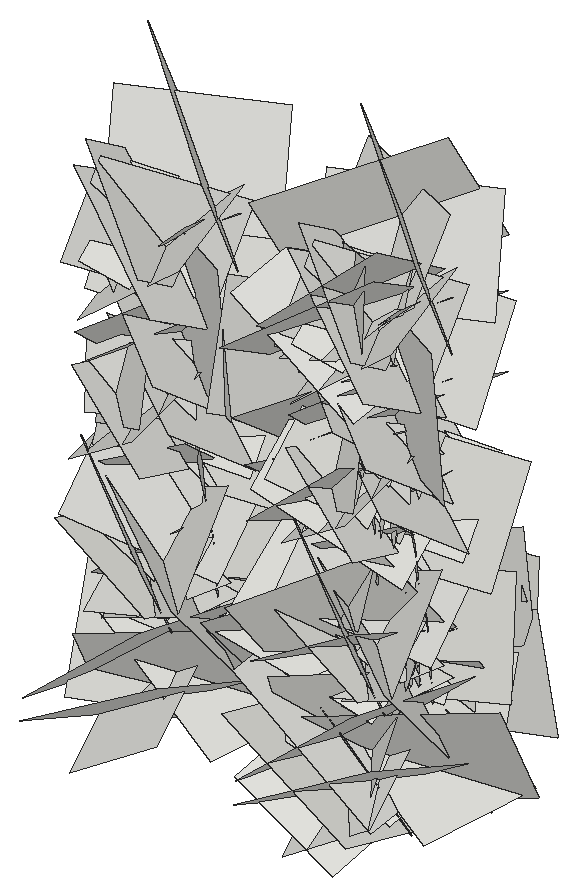
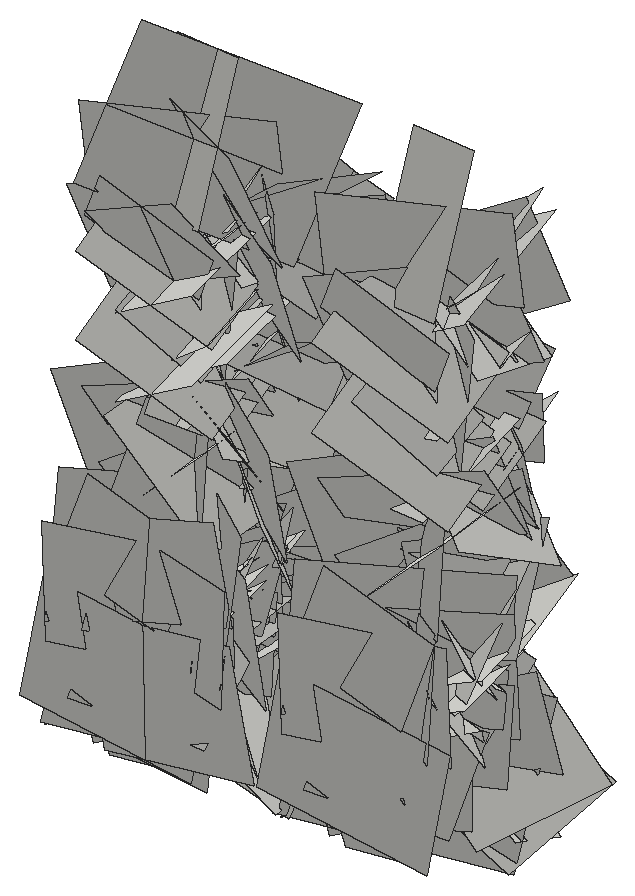
# SketchUp Ruby script. Lengths in inches.
U = 1.inch
M = Sketchup.active_model
def pt(a) = Geom::Point3d.new(a.map { |v| v * U })
def face(e, loops, mat)
  f = e.add_face(loops[0].map { |a| pt(a) })
  loops[1..].each { |l| e.add_face(l.map { |a| pt(a) }).erase! }
  f.material = f.back_material = mat if mat
  f
end
# faces: each face lists its corners as indices into pts; further lists are holes
def faces(e, pts, list, mat = nil) = list.each { |f| face(e, (f[0].is_a?(Array) ? f : [f]).map { |l| l.map { |i| pts[i] } }, mat) }
# xy, xz, yz: faces in a plane at the given z, y or x. An outline is a flat list of corners, or four numbers for a rectangle; further outlines are holes
def ring(l) = l.size == 4 ? [[l[0], l[1]], [l[2], l[1]], [l[2], l[3]], [l[0], l[3]]] : l.each_slice(2).to_a
def flat(e, list, mat, &to3) = list.each { |f| face(e, (f[0].is_a?(Array) ? f : [f]).map { |l| ring(l).map { |u, v| to3.(u, v) } }, mat) }
def xy(e, z, list, mat = nil) = flat(e, list, mat) { |x, y| [x, y, z] }
def xz(e, y, list, mat = nil) = flat(e, list, mat) { |x, z| [x, y, z] }
def yz(e, x, list, mat = nil) = flat(e, list, mat) { |y, z| [x, y, z] }
def lines(e, pts, list) = list.each { |a, b| e.add_line(pt(pts[a]), pt(pts[b])) }
# prism: a flat outline (further loops are holes) pulled along v
def prism(e, loops, v, mat = nil)
  f = face(e, loops, mat); d = Geom::Vector3d.new(v.map { |x| x * U })
  f.pushpull(f.normal.samedirection?(d) ? d.length : -d.length)
end
def box(e, o, s, mat = nil) = prism(e, [[o, [o[0] + s[0], o[1], o[2]], [o[0] + s[0], o[1] + s[1], o[2]], [o[0], o[1] + s[1], o[2]]]], [0, 0, s[2]], mat)
def at(x, y, z, deg = 0) = Geom::Transformation.translation(pt([x, y, z])) * Geom::Transformation.rotation(ORIGIN, Z_AXIS, deg.degrees)
def axes(o, x, y, z) = Geom::Transformation.new([*x, 0, *y, 0, *z, 0, *pt(o).to_a, 1])
def part(name) = M.definitions.add(name)
# library, detail: a bought-in or finely detailed component or shape, given as its bounding box
def library(name, o, s) = part(name).tap { |d| box(d.entities, o, s) }
def detail(e, o, s) = box(e.add_group.entities, o, s)
def put(e, d, t, mat = nil) = e.add_instance(d, t).tap { |i| i.material = mat if mat }
def group(e, t, mat = nil) = e.add_group.tap { |g| g.transformation = t; g.material = mat if mat }.entities
root = M.entities
c1 = part("Component\#6")
p = [[0.01,0,0],[0,3.24,4.54],[4.32,3.24,4.54],[4.33,0,0]]
faces(c1.entities,p,[[0,1,2,3]])
put(root,c1,axes([424.49,208.64,6.82],[-0.0498,0.28937,-0.67344],[-0.06797,-0.67386,-0.28508],[-0.77398,0.04056,0.06836]))
put(root,c1,axes([410.71,210.125,0.49],[0.19083,-0.77607,-0.35788],[0.04853,-0.35645,0.796],[0.90459,0.18284,0.03279]))
put(root,c1,axes([424.49,210.125,0.49],[-0.19083,-0.77607,-0.35788],[-0.04853,-0.35645,0.796],[-0.90459,0.18284,0.03279]))
put(root,c1,axes([420.52,210.125,0.49],[0.19083,-0.77607,-0.35788],[0.04853,-0.35645,0.796],[0.90459,0.18284,0.03279]))
put(root,c1,axes([410.71,210.53,-0.53],[-0.13793,-1.11303,0.36033],[0.12678,0.348,1.11812],[1.23359,-0.16021,-0.07463]))
put(root,c1,axes([424.49,210.53,-0.53],[0.13793,-1.11303,0.36033],[-0.12678,0.348,1.11812],[-1.23359,-0.16021,-0.07463]))
put(root,c1,axes([420.52,210.53,-0.53],[-0.13793,-1.11303,0.36033],[0.12678,0.348,1.11812],[1.23359,-0.16021,-0.07463]))
put(root,c1,axes([410.71,209.89,15.21],[0.14915,-0.31655,-0.61374],[0.00846,-0.62556,0.32448],[0.73195,0.07174,0.12131]))
put(root,c1,axes([424.49,209.89,15.21],[-0.14915,-0.31655,-0.61374],[-0.00846,-0.62556,0.32448],[-0.73195,0.07174,0.12131]))
put(root,c1,axes([420.52,209.89,15.21],[0.14915,-0.31655,-0.61374],[0.00846,-0.62556,0.32448],[0.73195,0.07174,0.12131]))
put(root,c1,axes([414.68,209.73,11.28],[0.10776,-0.78869,0.28769],[0.10217,0.29884,0.7852],[-0.88401,-0.0616,0.12582]))
put(root,c1,axes([420.52,209.73,11.28],[-0.10776,-0.78869,0.28769],[-0.10217,0.29884,0.7852],[0.88401,-0.0616,0.12582]))
put(root,c1,axes([424.49,209.73,11.28],[0.10776,-0.78869,0.28769],[0.10217,0.29884,0.7852],[-0.88401,-0.0616,0.12582]))
put(root,c1,axes([424.49,208.44,11.85],[0.18719,0.63062,-0.8853],[0.07209,-0.90156,-0.62864],[-1.1499,0.04614,-0.18352]))
put(root,c1,axes([410.71,208.44,11.85],[-0.18719,0.63062,-0.8853],[-0.07209,-0.90156,-0.62864],[1.1499,0.04614,-0.18352]))
put(root,c1,axes([420.52,208.44,11.85],[-0.18719,0.63062,-0.8853],[-0.07209,-0.90156,-0.62864],[1.1499,0.04614,-0.18352]))
put(root,c1,axes([410.71,206.93,9.09],[-0.09893,0.82066,-0.28112],[0.08874,-0.2729,-0.82446],[0.91523,0.11517,0.04956]))
put(root,c1,axes([424.49,206.93,9.09],[0.09893,0.82066,-0.28112],[-0.08874,-0.2729,-0.82446],[-0.91523,0.11517,0.04956]))
put(root,c1,axes([420.52,206.93,9.09],[-0.09893,0.82066,-0.28112],[0.08874,-0.2729,-0.82446],[0.91523,0.11517,0.04956]))
put(root,c1,axes([414.68,210.2,16.34],[0.08816,-0.12898,-0.67949],[-0.09646,-0.68047,0.11803],[-0.72675,0.07467,-0.09809]))
put(root,c1,axes([420.52,210.2,16.34],[-0.08816,-0.12898,-0.67949],[0.09646,-0.68047,0.11803],[0.72675,0.07467,-0.09809]))
put(root,c1,axes([424.49,210.2,16.34],[0.08816,-0.12898,-0.67949],[-0.09646,-0.68047,0.11803],[-0.72675,0.07467,-0.09809]))
put(root,c1,axes([414.68,208.78,18.92],[-0.08317,0.53287,-0.42892],[0.0846,-0.42165,-0.53844],[-0.72013,-0.11108,-0.01372]))
put(root,c1,axes([420.52,208.78,18.92],[0.08317,0.53287,-0.42892],[-0.0846,-0.42165,-0.53844],[0.72013,-0.11108,-0.01372]))
put(root,c1,axes([424.49,208.78,18.92],[-0.08317,0.53287,-0.42892],[0.0846,-0.42165,-0.53844],[-0.72013,-0.11108,-0.01372]))
put(root,c1,axes([410.71,212.18,1.04],[-0.25647,-1.30664,0.09966],[-0.13645,0.12456,1.32049],[1.38234,-0.23013,0.14883]))
put(root,c1,axes([424.49,212.18,1.04],[0.25647,-1.30664,0.09966],[0.13645,0.12456,1.32049],[-1.38234,-0.23013,0.14883]))
put(root,c1,axes([420.52,212.18,1.04],[-0.25647,-1.30664,0.09966],[-0.13645,0.12456,1.32049],[1.38234,-0.23013,0.14883]))
put(root,c1,axes([410.71,208.07,23.15],[0.06368,1.0247,-0.55961],[-0.10104,-0.55418,-1.02498],[1.23347,-0.0983,-0.05507]))
put(root,c1,axes([424.49,208.07,23.15],[-0.06368,1.0247,-0.55961],[0.10104,-0.55418,-1.02498],[-1.23347,-0.0983,-0.05507]))
put(root,c1,axes([420.52,208.07,23.15],[0.06368,1.0247,-0.55961],[-0.10104,-0.55418,-1.02498],[1.23347,-0.0983,-0.05507]))
put(root,c1,axes([414.68,211.39,19.29],[0.15412,-0.67583,-0.24542],[-0.06417,-0.26101,0.68288],[-0.75944,-0.11509,-0.10751]))
put(root,c1,axes([420.52,211.39,19.29],[-0.15412,-0.67583,-0.24542],[0.06417,-0.26101,0.68288],[0.75944,-0.11509,-0.10751]))
put(root,c1,axes([424.49,211.39,19.29],[0.15412,-0.67583,-0.24542],[-0.06417,-0.26101,0.68288],[-0.75944,-0.11509,-0.10751]))
put(root,c1,axes([414.68,210.2,18.35],[0.0434,-0.8468,0.50557],[0.21084,0.5027,0.82588],[-1.02393,0.06762,0.19149]))
put(root,c1,axes([420.52,210.2,18.35],[-0.0434,-0.8468,0.50557],[-0.21084,0.5027,0.82588],[1.02393,0.06762,0.19149]))
put(root,c1,axes([424.49,210.2,18.35],[0.0434,-0.8468,0.50557],[0.21084,0.5027,0.82588],[-1.02393,0.06762,0.19149]))
put(root,c1,axes([410.71,211.18,6.7],[0.06152,-0.66215,-0.45123],[0.20693,-0.42709,0.65185],[0.82377,0.15673,-0.13005]))
put(root,c1,axes([424.49,211.18,6.7],[-0.06152,-0.66215,-0.45123],[-0.20693,-0.42709,0.65185],[-0.82377,0.15673,-0.13005]))
put(root,c1,axes([420.52,211.18,6.7],[0.06152,-0.66215,-0.45123],[0.20693,-0.42709,0.65185],[0.82377,0.15673,-0.13005]))
put(root,c1,axes([410.71,209.17,10.9],[-0.01303,0.87895,-0.98683],[-0.04513,-0.98662,-0.87824],[1.40007,-0.02362,-0.03749]))
put(root,c1,axes([424.49,209.17,10.9],[0.01303,0.87895,-0.98683],[0.04513,-0.98662,-0.87824],[-1.40007,-0.02362,-0.03749]))
put(root,c1,axes([420.52,209.17,10.9],[-0.01303,0.87895,-0.98683],[-0.04513,-0.98662,-0.87824],[1.40007,-0.02362,-0.03749]))
put(root,c1,axes([410.71,212.1,18.5625],[0.14567,-1.06407,-0.312],[-0.08976,-0.32354,1.06612],[1.17197,0.10748,0.12044]))
put(root,c1,axes([424.49,212.1,18.5625],[-0.14567,-1.06407,-0.312],[0.08976,-0.32354,1.06612],[-1.17197,0.10748,0.12044]))
put(root,c1,axes([420.52,212.1,18.5625],[0.14567,-1.06407,-0.312],[-0.08976,-0.32354,1.06612],[1.17197,0.10748,0.12044]))
put(root,c1,axes([410.71,212.58,7.86],[0.11208,-0.8157,-0.84783],[-0.04176,-0.85323,0.81597],[1.2464,0.04476,0.10358]))
put(root,c1,axes([424.49,212.58,7.86],[-0.11208,-0.8157,-0.84783],[0.04176,-0.85323,0.81597],[-1.2464,0.04476,0.10358]))
put(root,c1,axes([420.52,212.58,7.86],[0.11208,-0.8157,-0.84783],[-0.04176,-0.85323,0.81597],[1.2464,0.04476,0.10358]))
put(root,c1,axes([410.71,213.11,12.64],[-0.17797,-1.01022,-0.50589],[-0.14692,-0.48916,1.02282],[1.18855,-0.21174,0.05069]))
put(root,c1,axes([424.49,213.11,12.64],[0.17797,-1.01022,-0.50589],[0.14692,-0.48916,1.02282],[-1.18855,-0.21174,0.05069]))
put(root,c1,axes([420.52,213.11,12.64],[-0.17797,-1.01022,-0.50589],[-0.14692,-0.48916,1.02282],[1.18855,-0.21174,0.05069]))
put(root,c1,axes([424.49,207.33,19.43],[-0.19308,0.28824,0.9525],[0.12727,0.96762,-0.26985],[-1.04716,0.06445,-0.20842]))
put(root,c1,axes([410.71,207.33,19.43],[0.19308,0.28824,0.9525],[-0.12727,0.96762,-0.26985],[1.04716,0.06445,-0.20842]))
put(root,c1,axes([420.52,207.33,19.43],[0.19308,0.28824,0.9525],[-0.12727,0.96762,-0.26985],[1.04716,0.06445,-0.20842]))
put(root,c1,axes([410.71,209.23,19.24],[0.2079,0.89177,-0.6436],[-0.06754,-0.64344,-0.91097],[1.16379,-0.19665,0.06211]))
put(root,c1,axes([424.49,209.23,19.24],[-0.2079,0.89177,-0.6436],[0.06754,-0.64344,-0.91097],[-1.16379,-0.19665,0.06211]))
put(root,c1,axes([420.52,209.23,19.24],[0.2079,0.89177,-0.6436],[-0.06754,-0.64344,-0.91097],[1.16379,-0.19665,0.06211]))
put(root,c1,axes([414.68,209.48,12.42],[-0.00847,0.47556,-0.37402],[-0.05873,-0.37306,-0.47315],[-0.63863,0.028,0.04848]))
put(root,c1,axes([420.52,209.48,12.42],[0.00847,0.47556,-0.37402],[0.05873,-0.37306,-0.47315],[0.63863,0.028,0.04848]))
put(root,c1,axes([424.49,209.48,12.42],[-0.00847,0.47556,-0.37402],[-0.05873,-0.37306,-0.47315],[-0.63863,0.028,0.04848]))
put(root,c1,axes([410.71,207.16,9.13],[0.13241,0.57393,0.92472],[-0.131,0.93225,-0.56191],[1.14619,0.04024,-0.17105]))
put(root,c1,axes([424.49,207.16,9.13],[-0.13241,0.57393,0.92472],[0.131,0.93225,-0.56191],[-1.14619,0.04024,-0.17105]))
put(root,c1,axes([420.52,207.16,9.13],[0.13241,0.57393,0.92472],[-0.131,0.93225,-0.56191],[1.14619,0.04024,-0.17105]))
put(root,c1,axes([410.71,212.32,20.17],[0.18703,-0.0568,-1.36224],[0.02248,-1.37332,0.06001],[1.44505,0.02871,0.17537]))
put(root,c1,axes([424.49,212.32,20.17],[-0.18703,-0.0568,-1.36224],[-0.02248,-1.37332,0.06001],[-1.44505,0.02871,0.17537]))
put(root,c1,axes([420.52,212.32,20.17],[0.18703,-0.0568,-1.36224],[0.02248,-1.37332,0.06001],[1.44505,0.02871,0.17537]))
put(root,c1,axes([414.68,211.74,12.76],[-0.12736,-0.0958,-0.74557],[0.10526,-0.75044,0.08042],[-0.78982,-0.08457,0.13094]))
put(root,c1,axes([420.52,211.74,12.76],[0.12736,-0.0958,-0.74557],[-0.10526,-0.75044,0.08042],[0.78982,-0.08457,0.13094]))
put(root,c1,axes([424.49,211.74,12.76],[-0.12736,-0.0958,-0.74557],[0.10526,-0.75044,0.08042],[-0.78982,-0.08457,0.13094]))
put(root,c1,axes([410.71,209.9375,16.21],[0.25577,0.83815,-0.61941],[0.04278,-0.64283,-0.85412],[1.10389,-0.16928,0.17662]))
put(root,c1,axes([424.49,209.9375,16.21],[-0.25577,0.83815,-0.61941],[-0.04278,-0.64283,-0.85412],[-1.10389,-0.16928,0.17662]))
put(root,c1,axes([420.52,209.9375,16.21],[0.25577,0.83815,-0.61941],[0.04278,-0.64283,-0.85412],[1.10389,-0.16928,0.17662]))
put(root,c1,axes([410.71,210.25,-0.65],[0.14226,-0.69765,1.16631],[0.2044,1.1699,0.67761],[1.42601,-0.0981,-0.21348]))
put(root,c1,axes([424.49,210.25,-0.65],[-0.14226,-0.69765,1.16631],[-0.2044,1.1699,0.67761],[-1.42601,-0.0981,-0.21348]))
put(root,c1,axes([420.52,210.25,-0.65],[0.14226,-0.69765,1.16631],[0.2044,1.1699,0.67761],[1.42601,-0.0981,-0.21348]))
put(root,c1,axes([424.49,208.82,8.26],[0.05727,0.78185,-0.16779],[-0.14528,-0.15663,-0.77398],[-0.83509,0.08087,0.12314]))
put(root,c1,axes([410.71,208.82,8.26],[-0.05727,0.78185,-0.16779],[0.14528,-0.15663,-0.77398],[0.83509,0.08087,0.12314]))
put(root,c1,axes([420.52,208.82,8.26],[-0.05727,0.78185,-0.16779],[0.14528,-0.15663,-0.77398],[0.83509,0.08087,0.12314]))
put(root,c1,axes([410.71,211.87,13.61],[0.09122,-0.87293,0.35057],[-0.03759,0.34878,0.87716],[0.99643,0.09307,0.001]))
put(root,c1,axes([424.49,211.87,13.61],[-0.09122,-0.87293,0.35057],[0.03759,0.34878,0.87716],[-0.99643,0.09307,0.001]))
put(root,c1,axes([420.52,211.87,13.61],[0.09122,-0.87293,0.35057],[-0.03759,0.34878,0.87716],[0.99643,0.09307,0.001]))
put(root,c1,axes([414.68,210.23,8.89],[-0.07411,0.69071,-0.39914],[0.11234,-0.38908,-0.69186],[-0.83811,-0.11323,-0.05744]))
put(root,c1,axes([420.52,210.23,8.89],[0.07411,0.69071,-0.39914],[-0.11234,-0.38908,-0.69186],[0.83811,-0.11323,-0.05744]))
put(root,c1,axes([424.49,210.23,8.89],[-0.07411,0.69071,-0.39914],[0.11234,-0.38908,-0.69186],[-0.83811,-0.11323,-0.05744]))
put(root,c1,axes([424.49,208.7,17.77],[-0.06939,0.44909,1.0594],[-0.12824,1.05255,-0.45366],[-1.21294,-0.13697,-0.01265]))
put(root,c1,axes([410.71,208.7,17.77],[0.06939,0.44909,1.0594],[0.12824,1.05255,-0.45366],[1.21294,-0.13697,-0.01265]))
put(root,c1,axes([420.52,208.7,17.77],[0.06939,0.44909,1.0594],[0.12824,1.05255,-0.45366],[1.21294,-0.13697,-0.01265]))
put(root,c1,axes([410.71,207.55,1.43],[-0.12288,0.50669,1.25804],[-0.22547,1.24021,-0.51911],[1.41983,0.2408,0.02645]))
put(root,c1,axes([424.49,207.55,1.43],[0.12288,0.50669,1.25804],[0.22547,1.24021,-0.51911],[-1.41983,0.2408,0.02645]))
put(root,c1,axes([420.52,207.55,1.43],[-0.12288,0.50669,1.25804],[-0.22547,1.24021,-0.51911],[1.41983,0.2408,0.02645]))
put(root,c1,axes([414.68,209.4375,21.31],[0.06259,0.84258,-0.05617],[0.1593,-0.0659,-0.83045],[-0.88082,0.04795,-0.15418]))
put(root,c1,axes([420.52,209.4375,21.31],[-0.06259,0.84258,-0.05617],[-0.1593,-0.0659,-0.83045],[0.88082,0.04795,-0.15418]))
put(root,c1,axes([424.49,209.4375,21.31],[0.06259,0.84258,-0.05617],[0.1593,-0.0659,-0.83045],[-0.88082,0.04795,-0.15418]))
put(root,c1,axes([424.49,209.66,7.46],[0.07333,0.81549,-0.13491],[-0.15326,-0.12136,-0.8077],[-0.86266,0.09088,0.13203]))
put(root,c1,axes([410.71,209.66,7.46],[-0.07333,0.81549,-0.13491],[0.15326,-0.12136,-0.8077],[0.86266,0.09088,0.13203]))
put(root,c1,axes([420.52,209.66,7.46],[-0.07333,0.81549,-0.13491],[0.15326,-0.12136,-0.8077],[0.86266,0.09088,0.13203]))
put(root,c1,axes([414.68,208.59,6.01],[0.08926,0.55811,0.79685],[0.15858,0.78289,-0.56414],[-1.01897,0.17073,-0.01799]))
put(root,c1,axes([420.52,208.59,6.01],[-0.08926,0.55811,0.79685],[-0.15858,0.78289,-0.56414],[1.01897,0.17073,-0.01799]))
put(root,c1,axes([424.49,208.59,6.01],[0.08926,0.55811,0.79685],[0.15858,0.78289,-0.56414],[-1.01897,0.17073,-0.01799]))
put(root,c1,axes([410.71,209.05,10.75],[0.11444,0.37825,1.13851],[0.07236,1.13932,-0.38499],[1.26962,-0.09903,-0.08068]))
put(root,c1,axes([424.49,209.05,10.75],[-0.11444,0.37825,1.13851],[-0.07236,1.13932,-0.38499],[-1.26962,-0.09903,-0.08068]))
put(root,c1,axes([420.52,209.05,10.75],[0.11444,0.37825,1.13851],[0.07236,1.13932,-0.38499],[1.26962,-0.09903,-0.08068]))
put(root,c1,axes([410.71,209.13,4.61],[0.2016,1.24111,0.06484],[-0.01549,0.06782,-1.25535],[1.31728,-0.18915,-0.02468]))
put(root,c1,axes([424.49,209.13,4.61],[-0.2016,1.24111,0.06484],[0.01549,0.06782,-1.25535],[-1.31728,-0.18915,-0.02468]))
put(root,c1,axes([420.52,209.13,4.61],[0.2016,1.24111,0.06484],[-0.01549,0.06782,-1.25535],[1.31728,-0.18915,-0.02468]))
put(root,c1,axes([414.68,210.26,8.16],[-0.03239,0.64464,-0.05696],[-0.08466,-0.06034,-0.64009],[-0.68073,-0.02317,0.08231]))
put(root,c1,axes([420.52,210.26,8.16],[0.03239,0.64464,-0.05696],[0.08466,-0.06034,-0.64009],[0.68073,-0.02317,0.08231]))
put(root,c1,axes([424.49,210.26,8.16],[-0.03239,0.64464,-0.05696],[-0.08466,-0.06034,-0.64009],[-0.68073,-0.02317,0.08231]))
put(root,c1,axes([410.71,212.31,27.23],[-0.13595,0.64817,-1.16375],[-0.16935,-1.16817,-0.63303],[1.40181,-0.07826,-0.18933]))
put(root,c1,axes([424.49,212.31,27.23],[0.13595,0.64817,-1.16375],[0.16935,-1.16817,-0.63303],[-1.40181,-0.07826,-0.18933]))
put(root,c1,axes([420.52,212.31,27.23],[-0.13595,0.64817,-1.16375],[-0.16935,-1.16817,-0.63303],[1.40181,-0.07826,-0.18933]))
put(root,c1,axes([410.71,209.54,11.71],[-0.0382,0.56931,0.80625],[0.18345,0.79793,-0.5557],[1.03,-0.121,0.12888]))
put(root,c1,axes([424.49,209.54,11.71],[0.0382,0.56931,0.80625],[-0.18345,0.79793,-0.5557],[-1.03,-0.121,0.12888]))
put(root,c1,axes([420.52,209.54,11.71],[-0.0382,0.56931,0.80625],[0.18345,0.79793,-0.5557],[1.03,-0.121,0.12888]))
put(root,c1,axes([410.71,210.59,2.66],[-0.04023,-0.02679,0.90097],[0.06825,0.89939,0.02945],[0.95301,-0.06554,0.03592]))
put(root,c1,axes([424.49,210.59,2.66],[0.04023,-0.02679,0.90097],[-0.06825,0.89939,0.02945],[-0.95301,-0.06554,0.03592]))
put(root,c1,axes([420.52,210.59,2.66],[-0.04023,-0.02679,0.90097],[0.06825,0.89939,0.02945],[0.95301,-0.06554,0.03592]))
put(root,c1,axes([414.68,210.86,7.98],[0.16776,-0.30988,0.90566],[0.16933,0.91363,0.28469],[-1.00041,0.10267,0.20006]))
put(root,c1,axes([420.52,210.86,7.98],[-0.16776,-0.30988,0.90566],[-0.16933,0.91363,0.28469],[1.00041,0.10267,0.20006]))
put(root,c1,axes([424.49,210.86,7.98],[0.16776,-0.30988,0.90566],[0.16933,0.91363,0.28469],[-1.00041,0.10267,0.20006]))
put(root,c1,axes([410.71,209.9375,13.64],[-0.01722,0.9911,-0.0782],[-0.18047,-0.07983,-0.97637],[1.03826,0.00256,-0.17101]))
put(root,c1,axes([424.49,209.9375,13.64],[0.01722,0.9911,-0.0782],[0.18047,-0.07983,-0.97637],[-1.03826,0.00256,-0.17101]))
put(root,c1,axes([420.52,209.9375,13.64],[-0.01722,0.9911,-0.0782],[-0.18047,-0.07983,-0.97637],[1.03826,0.00256,-0.17101]))
put(root,c1,axes([424.49,209.74,20.23],[0.19527,0.38459,1.04089],[-0.21918,1.04855,-0.35083],[-1.15564,-0.13388,0.24241]))
put(root,c1,axes([410.71,209.74,20.23],[-0.19527,0.38459,1.04089],[0.21918,1.04855,-0.35083],[1.15564,-0.13388,0.24241]))
put(root,c1,axes([420.52,209.74,20.23],[-0.19527,0.38459,1.04089],[0.21918,1.04855,-0.35083],[1.15564,-0.13388,0.24241]))
put(root,c1,axes([410.71,209.94,4.23],[-0.07499,0.16237,1.17608],[0.09639,1.17545,-0.15681],[1.25477,-0.08059,0.08234]))
put(root,c1,axes([424.49,209.94,4.23],[0.07499,0.16237,1.17608],[-0.09639,1.17545,-0.15681],[-1.25477,-0.08059,0.08234]))
put(root,c1,axes([420.52,209.94,4.23],[-0.07499,0.16237,1.17608],[0.09639,1.17545,-0.15681],[1.25477,-0.08059,0.08234]))
put(root,c1,axes([414.68,211.25,18.13],[-0.01725,0.58763,-0.23192],[0.06908,-0.2292,-0.5853],[-0.66607,-0.03899,-0.0547]))
put(root,c1,axes([420.52,211.25,18.13],[0.01725,0.58763,-0.23192],[-0.06908,-0.2292,-0.5853],[0.66607,-0.03899,-0.0547]))
put(root,c1,axes([424.49,211.25,18.13],[-0.01725,0.58763,-0.23192],[0.06908,-0.2292,-0.5853],[-0.66607,-0.03899,-0.0547]))
put(root,c1,axes([414.68,210.82,6.78],[-0.05791,0.63342,0.22945],[-0.07755,0.22326,-0.63376],[-0.7099,-0.07606,0.05052]))
put(root,c1,axes([424.49,210.82,6.78],[-0.05791,0.63342,0.22945],[-0.07755,0.22326,-0.63376],[-0.7099,-0.07606,0.05052]))
put(root,c1,axes([420.52,210.82,6.78],[0.05791,0.63342,0.22945],[0.07755,0.22326,-0.63376],[0.7099,-0.07606,0.05052]))
put(root,c1,axes([410.71,213.68,13.61],[0.09122,-0.87293,0.35057],[-0.03759,0.34878,0.87716],[0.99643,0.09307,0.001]))
put(root,c1,axes([410.71,213.68,16.94],[0.09122,-0.87293,0.35057],[-0.03759,0.34878,0.87716],[0.99643,0.09307,0.001]))
put(root,c1,axes([424.49,213.68,13.61],[-0.09122,-0.87293,0.35057],[0.03759,0.34878,0.87716],[-0.99643,0.09307,0.001]))
put(root,c1,axes([424.49,213.68,16.94],[-0.09122,-0.87293,0.35057],[0.03759,0.34878,0.87716],[-0.99643,0.09307,0.001]))
put(root,c1,axes([420.52,213.68,13.61],[0.09122,-0.87293,0.35057],[-0.03759,0.34878,0.87716],[0.99643,0.09307,0.001]))
put(root,c1,axes([420.52,213.68,16.94],[0.09122,-0.87293,0.35057],[-0.03759,0.34878,0.87716],[0.99643,0.09307,0.001]))
put(root,c1,axes([410.71,210.81,4.97],[0.03332,-0.20638,1.23099],[-0.11506,1.22627,0.20836],[1.31805,0.11226,-0.01293]))
put(root,c1,axes([424.49,210.81,4.97],[-0.03332,-0.20638,1.23099],[0.11506,1.22627,0.20836],[-1.31805,0.11226,-0.01293]))
put(root,c1,axes([420.52,210.81,4.97],[0.03332,-0.20638,1.23099],[-0.11506,1.22627,0.20836],[1.31805,0.11226,-0.01293]))
put(root,c1,axes([414.68,213.28,4.19],[-0.08194,0.11028,-0.62172],[-0.07302,-0.6241,-0.10214],[-0.66532,0.05491,0.08778]))
put(root,c1,axes([420.52,213.28,4.19],[0.08194,0.11028,-0.62172],[0.07302,-0.6241,-0.10214],[0.66532,0.05491,0.08778]))
put(root,c1,axes([424.49,213.28,4.19],[-0.08194,0.11028,-0.62172],[-0.07302,-0.6241,-0.10214],[-0.66532,0.05491,0.08778]))
put(root,c1,axes([414.68,211.49,4.24],[0.12406,-0.24562,0.96087],[0.14629,0.96216,0.22914],[-1.04104,0.10594,0.1467]))
put(root,c1,axes([420.52,211.49,4.24],[-0.12406,-0.24562,0.96087],[-0.14629,0.96216,0.22914],[1.04104,0.10594,0.1467]))
put(root,c1,axes([424.49,211.49,4.24],[0.12406,-0.24562,0.96087],[0.14629,0.96216,0.22914],[-1.04104,0.10594,0.1467]))
put(root,c1,axes([410.71,213.625,2.08],[0.05814,-0.55559,0.66869],[0.23916,0.65616,0.52668],[0.88998,-0.14003,-0.18522]))
put(root,c1,axes([424.49,213.625,2.08],[-0.05814,-0.55559,0.66869],[-0.23916,0.65616,0.52668],[-0.88998,-0.14003,-0.18522]))
put(root,c1,axes([420.52,213.625,2.08],[0.05814,-0.55559,0.66869],[0.23916,0.65616,0.52668],[0.88998,-0.14003,-0.18522]))
put(root,c1,axes([410.04,214.43,20.82],[0.40689,-0.33066,-0.61889],[0.38957,-0.50621,0.4984],[0.63361,0.52358,0.09101]))
put(root,c1,axes([425.17,214.43,20.82],[-0.40689,-0.33066,-0.61889],[-0.38957,-0.50621,0.4984],[-0.63361,0.52358,0.09101]))
put(root,c1,axes([419.84,214.43,20.82],[0.40689,-0.33066,-0.61889],[0.38957,-0.50621,0.4984],[0.63361,0.52358,0.09101]))
put(root,c1,axes([415.26,214.33,3.125],[-0.1239,-0.08914,-0.58356],[-0.39991,-0.44626,0.14373],[-0.48128,0.39377,0.0308]))
put(root,c1,axes([419.95,214.33,3.125],[0.1239,-0.08914,-0.58356],[0.39991,-0.44626,0.14373],[0.48128,0.39377,0.0308]))
put(root,c1,axes([425.06,214.33,3.125],[-0.1239,-0.08914,-0.58356],[-0.39991,-0.44626,0.14373],[-0.48128,0.39377,0.0308]))
put(root,c1,axes([410.56,213.9375,9.46],[-0.03176,-0.01156,-1.03134],[0.82675,-0.67538,-0.01509],[0.71538,0.78001,-0.02835]))
put(root,c1,axes([424.65,213.9375,9.46],[0.03176,-0.01156,-1.03134],[-0.82675,-0.67538,-0.01509],[-0.71538,0.78001,-0.02835]))
put(root,c1,axes([420.36,213.9375,9.46],[-0.03176,-0.01156,-1.03134],[0.82675,-0.67538,-0.01509],[0.71538,0.78001,-0.02835]))
put(root,c1,axes([415.31,214.375,11.05],[0.24885,0.08416,-0.78609],[-0.48118,-0.65702,-0.20591],[-0.6861,0.4913,-0.14071]))
put(root,c1,axes([419.9,214.375,11.05],[-0.24885,0.08416,-0.78609],[0.48118,-0.65702,-0.20591],[0.6861,0.4913,-0.14071]))
put(root,c1,axes([425.11,214.375,11.05],[0.24885,0.08416,-0.78609],[-0.48118,-0.65702,-0.20591],[-0.6861,0.4913,-0.14071]))
put(root,c1,axes([409.9,214.56,5.98],[0.23258,-0.01173,-1.12749],[0.77314,-0.87447,0.15104],[0.91146,0.74476,0.15959]))
put(root,c1,axes([425.3,214.56,5.98],[-0.23258,-0.01173,-1.12749],[-0.77314,-0.87447,0.15104],[-0.91146,0.74476,0.15959]))
put(root,c1,axes([419.71,214.56,5.98],[0.23258,-0.01173,-1.12749],[0.77314,-0.87447,0.15104],[0.91146,0.74476,0.15959]))
